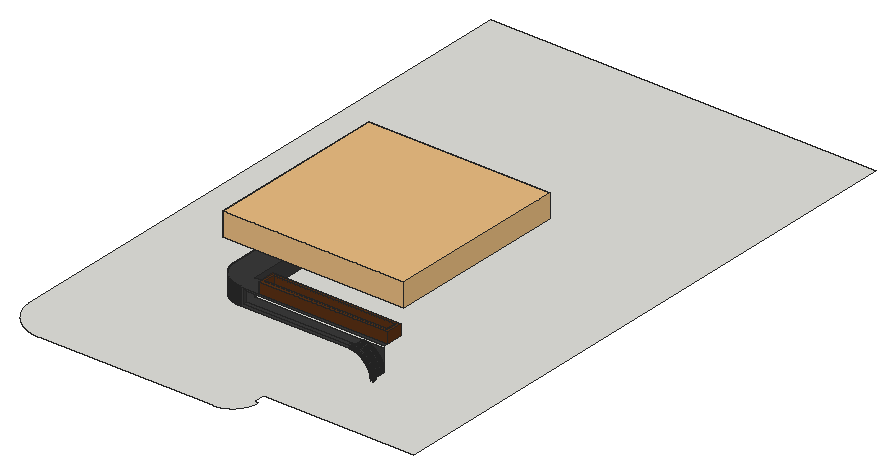
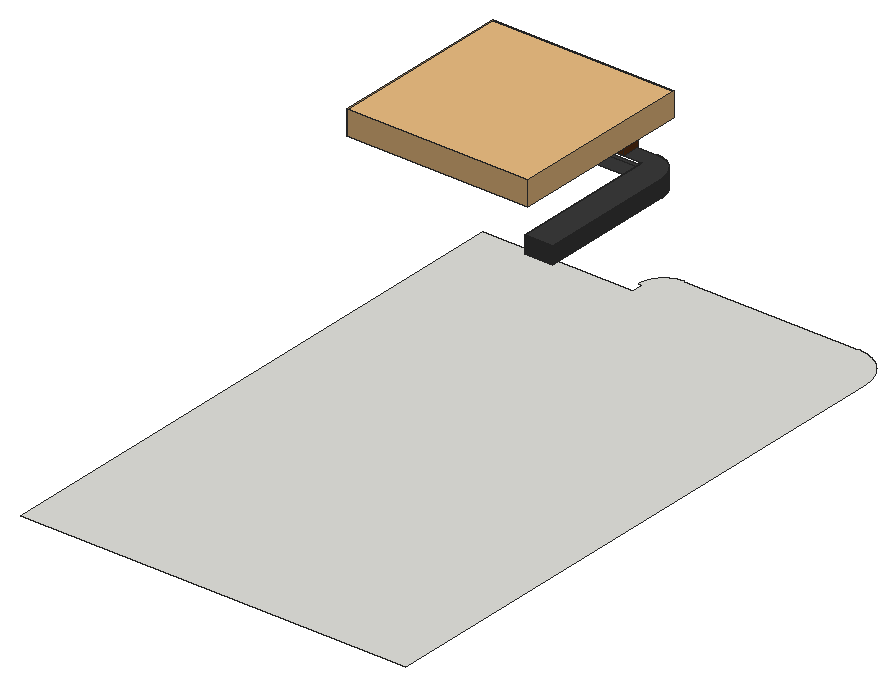
# SketchUp Ruby script. Lengths in inches.
U = 1.inch
M = Sketchup.active_model
def pt(a) = Geom::Point3d.new(a.map { |v| v * U })
def face(e, loops, mat)
  f = e.add_face(loops[0].map { |a| pt(a) })
  loops[1..].each { |l| e.add_face(l.map { |a| pt(a) }).erase! }
  f.material = f.back_material = mat if mat
  f
end
# faces: each face lists its corners as indices into pts; further lists are holes
def faces(e, pts, list, mat = nil) = list.each { |f| face(e, (f[0].is_a?(Array) ? f : [f]).map { |l| l.map { |i| pts[i] } }, mat) }
# xy, xz, yz: faces in a plane at the given z, y or x. An outline is a flat list of corners, or four numbers for a rectangle; further outlines are holes
def ring(l) = l.size == 4 ? [[l[0], l[1]], [l[2], l[1]], [l[2], l[3]], [l[0], l[3]]] : l.each_slice(2).to_a
def flat(e, list, mat, &to3) = list.each { |f| face(e, (f[0].is_a?(Array) ? f : [f]).map { |l| ring(l).map { |u, v| to3.(u, v) } }, mat) }
def xy(e, z, list, mat = nil) = flat(e, list, mat) { |x, y| [x, y, z] }
def xz(e, y, list, mat = nil) = flat(e, list, mat) { |x, z| [x, y, z] }
def yz(e, x, list, mat = nil) = flat(e, list, mat) { |y, z| [x, y, z] }
def lines(e, pts, list) = list.each { |a, b| e.add_line(pt(pts[a]), pt(pts[b])) }
# prism: a flat outline (further loops are holes) pulled along v
def prism(e, loops, v, mat = nil)
  f = face(e, loops, mat); d = Geom::Vector3d.new(v.map { |x| x * U })
  f.pushpull(f.normal.samedirection?(d) ? d.length : -d.length)
end
def box(e, o, s, mat = nil) = prism(e, [[o, [o[0] + s[0], o[1], o[2]], [o[0] + s[0], o[1] + s[1], o[2]], [o[0], o[1] + s[1], o[2]]]], [0, 0, s[2]], mat)
def at(x, y, z, deg = 0) = Geom::Transformation.translation(pt([x, y, z])) * Geom::Transformation.rotation(ORIGIN, Z_AXIS, deg.degrees)
def axes(o, x, y, z) = Geom::Transformation.new([*x, 0, *y, 0, *z, 0, *pt(o).to_a, 1])
def part(name) = M.definitions.add(name)
# library, detail: a bought-in or finely detailed component or shape, given as its bounding box
def library(name, o, s) = part(name).tap { |d| box(d.entities, o, s) }
def detail(e, o, s) = box(e.add_group.entities, o, s)
def put(e, d, t, mat = nil) = e.add_instance(d, t).tap { |i| i.material = mat if mat }
def group(e, t, mat = nil) = e.add_group.tap { |g| g.transformation = t; g.material = mat if mat }.entities
root = M.entities
M.materials.add("1496 AP 8293 CARBON COPY").color = [58, 58, 58]
M.materials.add("[Wood Cherry Original]").color = [91, 49, 20]
c1 = library("Group\#14",[-14,-14.57,-7.55],[148,148.57,19.55])
xy(root,273,[[43.57,64,185.27,64,185.55,64.01,185.82,64.02,186.1,64.03,186.375,64.04,186.65,64.06,186.92,64.09,187.2,64.12,187.74,64.18,188.01,64.22,188.29,64.26,188.56,64.3,189.1,64.4,189.37,64.46,189.63,64.52,189.9,64.58,190.44,64.72,190.96,64.86,191.23,64.94,191.49,65.03,191.75,65.11,192.01,65.2,192.27,65.3,192.53,65.39,192.78,65.49,193.04,65.6,193.79,65.93,194.29,66.17,194.53,66.29,194.78,66.42,195.02,66.54,195.26,66.68,195.5,66.8125,195.74,66.95,195.97,67.09,196.21,67.24,196.4375,67.39,196.67,67.54,196.89,67.69,197.12,67.85,197.56,68.17,198.22,68.68,198.43,68.85,198.85,69.21,199.05,69.39,199.25,69.58,199.46,69.77,199.65,69.96,199.85,70.15,200.04,70.35,200.23,70.54,200.42,70.75,200.61,70.95,200.79,71.15,201.15,71.57,201.32,71.78,201.83,72.44,202.15,72.88,202.31,73.11,202.46,73.33,202.61,73.5625,202.76,73.79,202.91,74.03,203.05,74.26,203.1875,74.5,203.32,74.74,203.46,74.98,203.58,75.22,203.71,75.47,203.83,75.71,204.07,76.21,204.4,76.96,204.51,77.22,204.61,77.47,204.7,77.73,204.8,77.99,204.89,78.25,204.97,78.51,205.06,78.77,205.14,79.04,205.28,79.56,205.42,80.1,205.48,80.37,205.54,80.63,205.6,80.9,205.7,81.44,205.74,81.71,205.78,81.99,205.82,82.26,205.88,82.8,205.91,83.08,205.94,83.35,205.96,83.625,205.97,83.9,205.98,84.18,205.99,84.45,206,84.73,206,85,203,85,203,94,326,94,326,567,11,567,11,96.57,11.01,96.14,11.03,95.7,11.07,94.84,11.1,94.41,11.18,93.55,11.28,92.69,11.34,92.26,11.41,91.84,11.48,91.41,11.55,90.99,11.63,90.5625,11.72,90.14,11.8125,89.72,11.91,89.3,12.02,88.875,12.125,88.46,12.24,88.04,12.36,87.63,12.48,87.21,12.62,86.8,12.75,86.39,12.89,85.98,13.04,85.58,13.19,85.17,13.51,84.37,13.68,83.97,13.85,83.58,14.03,83.18,14.21,82.79,14.4,82.4,14.6,82.02,14.8,81.63,15,81.25,15.42,80.5,15.86,79.76,16.09,79.39,16.32,79.03,16.5625,78.67,16.8,78.31,17.05,77.95,17.3,77.6,17.56,77.26,17.82,76.91,18.08,76.57,18.35,76.23,18.91,75.57,19.1875,75.24,19.48,74.92,19.77,74.6,20.0625,74.28,20.36,73.97,20.67,73.67,20.97,73.36,21.28,73.0625,21.6,72.77,21.92,72.48,22.24,72.1875,22.57,71.91,23.23,71.35,23.57,71.08,23.91,70.82,24.26,70.56,24.6,70.3,24.95,70.05,25.31,69.8,25.67,69.5625,26.03,69.32,26.39,69.09,26.76,68.86,27.5,68.42,28.25,68,28.63,67.8,29.02,67.6,29.4,67.4,29.79,67.21,30.18,67.03,30.58,66.85,30.97,66.68,31.37,66.51,32.17,66.19,32.58,66.04,32.98,65.89,33.39,65.75,33.8,65.62,34.21,65.48,34.63,65.36,35.04,65.24,35.46,65.125,35.875,65.02,36.3,64.91,36.72,64.8125,37.14,64.72,37.5625,64.63,37.99,64.55,38.41,64.48,38.84,64.41,39.26,64.34,39.69,64.28,40.55,64.18,41.41,64.1,41.84,64.07,42.7,64.03,43.14,64.01]])
xy(root,348.99,[[291.47,71,291.71,85]],"1496 AP 8293 CARBON COPY")
xy(root,349,[[202.76,71,202.52,71.01,202.28,71.01,201.8,71.03,201.56,71.05,201.32,71.0625,201.08,71.08,200.84,71.1,200.36,71.15,199.88,71.21,199.64,71.25,199.4,71.28,199.16,71.32,198.93,71.36,198.69,71.41,198.45,71.45,198.22,71.5,197.98,71.55,197.75,71.61,197.51,71.66,197.05,71.78,196.81,71.85,196.58,71.91,196.12,72.05,195.66,72.2,195.4375,72.28,195.21,72.36,194.98,72.44,194.76,72.53,194.53,72.62,194.31,72.7,194.09,72.8,193.87,72.89,193.43,73.09,193.21,73.1875,192.99,73.29,192.77,73.4,192.56,73.51,192.34,73.62,191.92,73.84,191.29,74.2,191.09,74.33,190.88,74.45,190.68,74.58,190.47,74.71,190.27,74.84,190.07,74.98,189.875,75.11,189.68,75.25,189.48,75.39,189.29,75.54,189.09,75.68,188.71,75.98,188.53,76.125,188.34,76.28,188.15,76.43,187.43,77.07,187.26,77.23,187.08,77.4,186.4,78.08,186.23,78.26,186.07,78.43,185.43,79.15,185.28,79.34,185.125,79.53,184.98,79.71,184.68,80.09,184.54,80.29,184.39,80.48,184.25,80.68,184.11,80.875,183.98,81.07,183.84,81.27,183.71,81.47,183.58,81.68,183.45,81.88,183.33,82.09,183.2,82.29,182.84,82.92,182.62,83.34,182.51,83.56,182.4,83.77,182.29,83.99,182.1875,84.21,182.09,84.43,181.89,84.87,181.8,85.09,181.7,85.31,181.62,85.53,181.53,85.76,181.44,85.98,181.36,86.21,181.28,86.4375,181.2,86.66,181.05,87.12,180.91,87.58,180.85,87.81,180.78,88.05,180.66,88.51,180.61,88.75,180.55,88.98,180.5,89.22,180.45,89.45,180.41,89.69,180.36,89.93,180.32,90.16,180.28,90.4,180.25,90.64,180.21,90.88,180.15,91.36,180.1,91.84,180.08,92.08,180.0625,92.32,180.05,92.56,180.03,92.8,180.01,93.28,180.01,93.52,180,93.76,180,205,203,205,203,85,291,85,291,71],[291,71,291.24,85]],"1496 AP 8293 CARBON COPY")
xy(root,351,[[205,71,291,74],[291,71,291.26,74]],"1496 AP 8293 CARBON COPY")
xy(root,361,[[205,71,321,74]],"1496 AP 8293 CARBON COPY")
xy(root,363,[[202.76,71,323,71,323,85,203,85,203,205,180,205,180,93.76,180.01,93.52,180.01,93.28,180.03,92.8,180.05,92.56,180.0625,92.32,180.08,92.08,180.1,91.84,180.15,91.36,180.21,90.88,180.25,90.64,180.28,90.4,180.32,90.16,180.36,89.93,180.41,89.69,180.45,89.45,180.5,89.22,180.55,88.98,180.61,88.75,180.66,88.51,180.78,88.05,180.85,87.81,180.91,87.58,181.05,87.12,181.2,86.66,181.28,86.4375,181.36,86.21,181.44,85.98,181.53,85.76,181.62,85.53,181.7,85.31,181.8,85.09,181.89,84.87,182.09,84.43,182.1875,84.21,182.29,83.99,182.4,83.77,182.51,83.56,182.62,83.34,182.84,82.92,183.2,82.29,183.33,82.09,183.45,81.88,183.58,81.68,183.71,81.47,183.84,81.27,183.98,81.07,184.11,80.875,184.25,80.68,184.39,80.48,184.54,80.29,184.68,80.09,184.98,79.71,185.125,79.53,185.28,79.34,185.43,79.15,186.07,78.43,186.23,78.26,186.4,78.08,187.08,77.4,187.26,77.23,187.43,77.07,188.15,76.43,188.34,76.28,188.53,76.125,188.71,75.98,189.09,75.68,189.29,75.54,189.48,75.39,189.68,75.25,189.875,75.11,190.07,74.98,190.27,74.84,190.47,74.71,190.68,74.58,190.88,74.45,191.09,74.33,191.29,74.2,191.92,73.84,192.34,73.62,192.56,73.51,192.77,73.4,192.99,73.29,193.21,73.1875,193.43,73.09,193.87,72.89,194.09,72.8,194.31,72.7,194.53,72.62,194.76,72.53,194.98,72.44,195.21,72.36,195.4375,72.28,195.66,72.2,196.12,72.05,196.58,71.91,196.81,71.85,197.05,71.78,197.51,71.66,197.75,71.61,197.98,71.55,198.22,71.5,198.45,71.45,198.69,71.41,198.93,71.36,199.16,71.32,199.4,71.28,199.64,71.25,199.88,71.21,200.36,71.15,200.84,71.1,201.08,71.08,201.32,71.0625,201.56,71.05,201.8,71.03,202.28,71.01,202.52,71.01]],"1496 AP 8293 CARBON COPY")
xz(root,71,[[202.76,349,203,363]],"1496 AP 8293 CARBON COPY")
xz(root,71.01,[[202.28,349,202.52,363]],"1496 AP 8293 CARBON COPY")
xz(root,85,[[309,331,309,331.24,308.99,331.47,308.99,331.71,308.98,331.94,308.96,332.18,308.94,332.41,308.92,332.65,308.9,332.88,308.875,333.12,308.85,333.35,308.8125,333.58,308.78,333.82,308.7,334.28,308.65,334.51,308.61,334.74,308.56,334.97,308.5,335.2,308.45,335.43,308.39,335.66,308.32,335.89,308.26,336.11,308.19,336.34,308.12,336.5625,308.04,336.79,307.97,337.01,307.89,337.23,307.8,337.45,307.72,337.67,307.54,338.11,307.44,338.32,307.35,338.54,307.25,338.75,307.14,338.96,307.04,339.17,306.82,339.59,306.7,339.8,306.59,340,306.35,340.4,306.22,340.61,306.1,340.8,305.97,341,305.83,341.2,305.7,341.39,305.5625,341.58,305.42,341.77,305.28,341.96,305.14,342.14,304.99,342.33,304.84,342.51,304.6875,342.69,304.53,342.87,304.375,343.04,304.22,343.22,304.06,343.39,303.89,343.56,303.73,343.73,303.56,343.89,303.39,344.06,303.22,344.22,303.04,344.375,302.87,344.53,302.69,344.6875,302.51,344.84,302.33,344.99,302.14,345.14,301.96,345.28,301.77,345.42,301.58,345.5625,301.39,345.7,301.2,345.83,301,345.97,300.8,346.1,300.61,346.22,300.4,346.35,300,346.59,299.8,346.7,299.59,346.82,299.17,347.04,298.96,347.14,298.75,347.25,298.54,347.35,298.32,347.44,298.11,347.54,297.67,347.72,297.45,347.8,297.23,347.89,297.01,347.97,296.79,348.04,296.5625,348.12,296.34,348.19,296.11,348.26,295.89,348.32,295.66,348.39,295.43,348.45,295.2,348.5,294.97,348.56,294.74,348.61,294.51,348.65,294.28,348.7,293.82,348.78,293.58,348.8125,293.35,348.85,293.12,348.875,292.88,348.9,292.65,348.92,292.41,348.94,292.18,348.96,291.94,348.98,291.71,348.99,291.47,348.99,291.24,349,291,349,309,349]],"1496 AP 8293 CARBON COPY")
xz(root,205,[[180,349,203,363]],"1496 AP 8293 CARBON COPY")
yz(root,180,[[93.76,349,94,363],[94,349,205,363]],"1496 AP 8293 CARBON COPY")
yz(root,180.01,[[93.28,349,93.52,363]],"1496 AP 8293 CARBON COPY")
yz(root,203,[[85,349,205,363]],"1496 AP 8293 CARBON COPY")
yz(root,205,[[71,351,74,361]],"1496 AP 8293 CARBON COPY")
yz(root,308.99,[[71,331.47,85,331.71]],"1496 AP 8293 CARBON COPY")
yz(root,309,[[71,331,85,331.24]],"1496 AP 8293 CARBON COPY")
yz(root,311,[[71,331,74,331.26]],"1496 AP 8293 CARBON COPY")
p = [[309,71,331.24],[308.99,71,331.47],[308.99,85,331.47],[309,85,331.24],[310.99,71,331.52],[311,71,331.26],
  [311,74,331.26],[310.99,74,331.52],[310.98,71,331.79],[310.98,74,331.79],[308.99,71,331.71],[308.98,71,331.94],
  [308.98,85,331.94],[308.99,85,331.71],[310.97,71,332.05],[310.97,74,332.05],[308.96,71,332.18],[308.96,85,332.18],
  [310.96,71,332.31],[310.96,74,332.31],[308.94,71,332.41],[308.94,85,332.41],[310.9375,71,332.57],[310.9375,74,332.57],
  [308.92,71,332.65],[308.92,85,332.65],[308.9,71,332.88],[308.9,85,332.88],[310.92,71,332.83],[310.92,74,332.83],
  [310.89,71,333.09],[310.89,74,333.09],[308.875,71,333.12],[308.875,85,333.12],[308.85,71,333.35],[308.85,85,333.35],
  [310.86,71,333.35],[310.86,74,333.35],[308.8125,71,333.58],[308.8125,85,333.58],[310.83,71,333.61],[310.83,74,333.61],
  [308.78,71,333.82],[308.78,85,333.82],[310.79,71,333.87],[310.79,74,333.87],[308.74,71,334.05],[308.74,85,334.05],
  [310.75,71,334.13],[310.75,74,334.13],[308.7,71,334.28],[308.7,85,334.28],[310.71,71,334.39],[310.71,74,334.39],
  [308.65,71,334.51],[308.65,85,334.51],[310.67,71,334.64],[310.67,74,334.64],[308.61,71,334.74],[308.61,85,334.74],
  [310.62,71,334.9],[310.62,74,334.9],[308.56,71,334.97],[308.56,85,334.97],[310.5625,71,335.16],[310.5625,74,335.16],
  [308.5,71,335.2],[308.5,85,335.2],[308.45,71,335.43],[308.45,85,335.43],[310.51,71,335.41],[310.51,74,335.41],
  [308.39,71,335.66],[308.39,85,335.66],[310.45,71,335.67],[310.45,74,335.67],[308.32,71,335.89],[308.32,85,335.89],
  [310.38,71,335.92],[310.38,74,335.92],[308.26,71,336.11],[308.26,85,336.11],[310.32,71,336.18],[310.32,74,336.18],
  [308.19,71,336.34],[308.19,85,336.34],[310.25,71,336.43],[310.25,74,336.43],[308.12,71,336.5625],[308.12,85,336.5625],
  [310.18,71,336.68],[310.18,74,336.68],[308.04,71,336.79],[308.04,85,336.79],[310.1,71,336.93],[310.1,74,336.93],
  [307.97,71,337.01],[307.97,85,337.01],[310.02,71,337.18],[310.02,74,337.18],[307.89,71,337.23],[307.89,85,337.23],
  [307.8,71,337.45],[307.8,85,337.45],[309.9375,71,337.43],[309.9375,74,337.43],[309.85,71,337.68],[309.85,74,337.68],
  [307.72,71,337.67],[307.72,85,337.67],[307.63,71,337.89],[307.63,85,337.89],[309.76,71,337.92],[309.76,74,337.92],
  [307.54,71,338.11],[307.54,85,338.11],[309.67,71,338.17],[309.67,74,338.17],[307.44,71,338.32],[307.44,85,338.32],
  [309.58,71,338.41],[309.58,74,338.41],[307.35,71,338.54],[307.35,85,338.54],[309.48,71,338.65],[309.48,74,338.65],
  [307.25,71,338.75],[307.25,85,338.75],[307.14,71,338.96],[307.14,85,338.96],[309.375,71,338.89],[309.375,74,338.89],
  [309.27,71,339.13],[309.27,74,339.13],[307.04,71,339.17],[307.04,85,339.17],[309.16,71,339.375],[309.16,74,339.375],
  [306.93,71,339.38],[306.93,85,339.38],[306.82,71,339.59],[306.82,85,339.59],[309.05,71,339.61],[309.05,74,339.61],
  [306.7,71,339.8],[306.7,85,339.8],[308.9375,71,339.85],[308.9375,74,339.85],[306.59,71,340],[306.59,85,340],
  [308.82,71,340.08],[308.82,74,340.08],[306.47,71,340.2],[306.47,85,340.2],[308.7,71,340.3125],[308.7,74,340.3125],
  [306.35,71,340.4],[306.35,85,340.4],[308.58,71,340.54],[308.58,74,340.54],[306.22,71,340.61],[306.22,85,340.61],
  [308.45,71,340.77],[308.45,74,340.77],[306.1,71,340.8],[306.1,85,340.8],[305.97,71,341],[305.97,85,341],
  [308.32,71,341],[308.32,74,341],[305.83,71,341.2],[305.83,85,341.2],[308.1875,71,341.23],[308.1875,74,341.23],
  [305.7,71,341.39],[305.7,85,341.39],[308.05,71,341.45],[308.05,74,341.45],[305.5625,71,341.58],[305.5625,85,341.58],
  [307.91,71,341.67],[307.91,74,341.67],[305.42,71,341.77],[305.42,85,341.77],[307.77,71,341.89],[307.77,74,341.89],
  [305.28,71,341.96],[305.28,85,341.96],[307.63,71,342.11],[307.63,74,342.11],[305.14,71,342.14],[305.14,85,342.14],
  [304.99,71,342.33],[304.99,85,342.33],[307.48,71,342.33],[307.48,74,342.33],[304.84,71,342.51],[304.84,85,342.51],
  [307.33,71,342.54],[307.33,74,342.54],[304.6875,71,342.69],[304.6875,85,342.69],[307.18,71,342.76],[307.18,74,342.76],
  [304.53,71,342.87],[304.53,85,342.87],[307.03,71,342.97],[307.03,74,342.97],[304.375,71,343.04],[304.375,85,343.04],
  [304.22,71,343.22],[304.22,85,343.22],[306.87,71,343.18],[306.87,74,343.18],[304.06,71,343.39],[304.06,85,343.39],
  [306.71,71,343.38],[306.71,74,343.38],[303.89,71,343.56],[303.89,85,343.56],[306.54,71,343.59],[306.54,74,343.59],
  [303.73,71,343.73],[303.73,85,343.73],[306.375,71,343.79],[306.375,74,343.79],[303.56,71,343.89],[303.56,85,343.89],
  [306.21,71,343.99],[306.21,74,343.99],[303.39,71,344.06],[303.39,85,344.06],[306.04,71,344.1875],[306.04,74,344.1875],
  [303.22,71,344.22],[303.22,85,344.22],[303.04,71,344.375],[303.04,85,344.375],[305.86,71,344.38],[305.86,74,344.38],
  [302.87,71,344.53],[302.87,85,344.53],[305.6875,71,344.58],[305.6875,74,344.58],[302.69,71,344.6875],[302.69,85,344.6875],
  [305.51,71,344.77],[305.51,74,344.77],[302.51,71,344.84],[302.51,85,344.84],[302.33,71,344.99],[302.33,85,344.99],
  [305.33,71,344.96],[305.33,74,344.96],[302.14,71,345.14],[302.14,85,345.14],[305.14,71,345.14],[305.14,74,345.14],
  [301.96,71,345.28],[301.96,85,345.28],[304.96,71,345.33],[304.96,74,345.33],[301.77,71,345.42],[301.77,85,345.42],
  [304.77,71,345.51],[304.77,74,345.51],[301.58,71,345.5625],[301.58,85,345.5625],[304.58,71,345.6875],[304.58,74,345.6875],
  [301.39,71,345.7],[301.39,85,345.7],[301.2,71,345.83],[301.2,85,345.83],[304.38,71,345.86],[304.38,74,345.86],
  [301,71,345.97],[301,85,345.97],[304.1875,71,346.04],[304.1875,74,346.04],[300.8,71,346.1],[300.8,85,346.1],
  [303.99,71,346.21],[303.99,74,346.21],[300.61,71,346.22],[300.61,85,346.22],[300.4,71,346.35],[300.4,85,346.35],
  [303.79,71,346.375],[303.79,74,346.375],[300.2,71,346.47],[300.2,85,346.47],[303.59,71,346.54],[303.59,74,346.54],
  [300,71,346.59],[300,85,346.59],[303.38,71,346.71],[303.38,74,346.71],[299.8,71,346.7],[299.8,85,346.7],
  [299.59,71,346.82],[299.59,85,346.82],[303.18,71,346.87],[303.18,74,346.87],[299.38,71,346.93],[299.38,85,346.93],
  [299.17,71,347.04],[299.17,85,347.04],[302.97,71,347.03],[302.97,74,347.03],[298.96,71,347.14],[298.96,85,347.14],
  [302.76,71,347.18],[302.76,74,347.18],[298.75,71,347.25],[298.75,85,347.25],[298.54,71,347.35],[298.54,85,347.35],
  [302.54,71,347.33],[302.54,74,347.33],[298.32,71,347.44],[298.32,85,347.44],[302.33,71,347.48],[302.33,74,347.48],
  [298.11,71,347.54],[298.11,85,347.54],[297.89,71,347.63],[297.89,85,347.63],[302.11,71,347.63],[302.11,74,347.63],
  [297.67,71,347.72],[297.67,85,347.72],[301.89,71,347.77],[301.89,74,347.77],[297.45,71,347.8],[297.45,85,347.8],
  [297.23,71,347.89],[297.23,85,347.89],[301.67,71,347.91],[301.67,74,347.91],[297.01,71,347.97],[297.01,85,347.97],
  [301.45,71,348.05],[301.45,74,348.05],[296.79,71,348.04],[296.5625,71,348.12],[296.5625,85,348.12],[296.79,85,348.04],
  [296.34,71,348.19],[296.34,85,348.19],[301.23,71,348.1875],[301.23,74,348.1875],[296.11,71,348.26],[296.11,85,348.26],
  [301,71,348.32],[301,74,348.32],[295.89,71,348.32],[295.66,71,348.39],[295.66,85,348.39],[295.89,85,348.32],
  [300.77,71,348.45],[300.77,74,348.45],[295.43,71,348.45],[295.2,71,348.5],[295.2,85,348.5],[295.43,85,348.45],
  [300.54,71,348.58],[300.54,74,348.58],[294.97,71,348.56],[294.97,85,348.56],[294.74,71,348.61],[294.51,71,348.65],
  [294.51,85,348.65],[294.74,85,348.61],[300.3125,71,348.7],[300.3125,74,348.7],[294.05,71,348.74],[293.82,71,348.78],
  [293.82,85,348.78],[294.05,85,348.74],[294.28,71,348.7],[294.28,85,348.7],[300.08,71,348.82],[300.08,74,348.82],
  [293.35,71,348.85],[293.12,71,348.875],[293.12,85,348.875],[293.35,85,348.85],[293.58,71,348.8125],[293.58,85,348.8125],
  [299.85,71,348.9375],[299.85,74,348.9375],[292.41,71,348.94],[292.18,71,348.96],[292.18,85,348.96],[292.41,85,348.94],
  [292.65,71,348.92],[292.65,85,348.92],[292.88,71,348.9],[292.88,85,348.9],[299.61,71,349.05],[299.61,74,349.05],
  [201.56,71.05,363],[201.32,71.0625,363],[201.32,71.0625,349],[201.56,71.05,349],[201.8,71.03,363],[201.8,71.03,349],
  [202.04,71.02,363],[202.04,71.02,349],[202.28,71.01,363],[202.28,71.01,349],[202.76,71,363],[202.52,71.01,363],
  [202.52,71.01,349],[202.76,71,349],[291.47,71,348.99],[291.24,71,349],[291.24,85,349],[291.47,85,348.99],
  [291.94,71,348.98],[291.71,71,348.99],[291.71,85,348.99],[291.94,85,348.98],[200.6,71.125,363],[200.36,71.15,363],
  [200.36,71.15,349],[200.6,71.125,349],[200.84,71.1,363],[200.84,71.1,349],[201.08,71.08,363],[201.08,71.08,349],
  [199.64,71.25,363],[199.4,71.28,363],[199.4,71.28,349],[199.64,71.25,349],[199.88,71.21,363],[199.88,71.21,349],
  [200.12,71.18,363],[200.12,71.18,349],[199.16,71.32,363],[198.93,71.36,363],[198.93,71.36,349],[199.16,71.32,349],
  [198.69,71.41,363],[198.45,71.45,363],[198.45,71.45,349],[198.69,71.41,349],[198.22,71.5,363],[197.98,71.55,363],
  [197.98,71.55,349],[198.22,71.5,349],[197.75,71.61,363],[197.51,71.66,363],[197.51,71.66,349],[197.75,71.61,349],
  [197.28,71.72,363],[197.05,71.78,363],[197.05,71.78,349],[197.28,71.72,349],[196.81,71.85,363],[196.58,71.91,363],
  [196.58,71.91,349],[196.81,71.85,349],[196.35,71.98,363],[196.35,71.98,349],[196.12,72.05,363],[196.12,72.05,349],
  [195.89,72.125,363],[195.66,72.2,363],[195.66,72.2,349],[195.89,72.125,349],[195.4375,72.28,363],[195.4375,72.28,349],
  [195.21,72.36,363],[195.21,72.36,349],[194.98,72.44,363],[194.76,72.53,363],[194.76,72.53,349],[194.98,72.44,349],
  [194.53,72.62,363],[194.53,72.62,349],[194.31,72.7,363],[194.31,72.7,349],[194.09,72.8,363],[194.09,72.8,349],
  [193.87,72.89,363],[193.87,72.89,349],[193.65,72.99,363],[193.65,72.99,349],[193.43,73.09,363],[193.43,73.09,349],
  [193.21,73.1875,363],[193.21,73.1875,349],[192.99,73.29,363],[192.99,73.29,349],[192.77,73.4,363],[192.77,73.4,349],
  [192.56,73.51,363],[192.56,73.51,349],[192.34,73.62,363],[192.34,73.62,349],[192.13,73.73,363],[192.13,73.73,349],
  [191.92,73.84,363],[191.92,73.84,349],[191.71,73.96,363],[191.71,73.96,349],[191.5,74.08,363],[191.5,74.08,349],
  [191.29,74.2,363],[191.29,74.2,349],[191.09,74.33,363],[191.09,74.33,349],[190.88,74.45,363],[190.88,74.45,349],
  [190.68,74.58,363],[190.68,74.58,349],[190.47,74.71,363],[190.47,74.71,349],[190.27,74.84,363],[190.27,74.84,349],
  [190.07,74.98,363],[190.07,74.98,349],[189.875,75.11,363],[189.875,75.11,349],[189.68,75.25,363],[189.68,75.25,349],
  [189.48,75.39,363],[189.48,75.39,349],[189.29,75.54,363],[189.29,75.54,349],[189.09,75.68,363],[189.09,75.68,349],
  [188.9,75.83,363],[188.9,75.83,349],[188.71,75.98,363],[188.71,75.98,349],[188.53,76.125,363],[188.53,76.125,349],
  [188.34,76.28,363],[188.34,76.28,349],[188.15,76.43,363],[188.15,76.43,349],[187.97,76.59,363],[187.97,76.59,349],
  [187.79,76.75,363],[187.79,76.75,349],[187.61,76.91,363],[187.61,76.91,349],[187.43,77.07,363],[187.43,77.07,349],
  [187.26,77.23,363],[187.26,77.23,349],[187.08,77.4,363],[187.08,77.4,349],[186.91,77.57,363],[186.91,77.57,349],
  [186.74,77.74,363],[186.74,77.74,349],[186.57,77.91,363],[186.57,77.91,349],[186.4,78.08,363],[186.4,78.08,349],
  [186.23,78.26,363],[186.23,78.26,349],[186.07,78.43,363],[186.07,78.43,349],[185.91,78.61,363],[185.91,78.61,349],
  [185.75,78.79,363],[185.75,78.79,349],[185.59,78.97,363],[185.59,78.97,349],[185.43,79.15,363],[185.43,79.15,349],
  [185.28,79.34,363],[185.28,79.34,349],[185.125,79.53,363],[185.125,79.53,349],[184.98,79.71,363],[184.98,79.71,349],
  [184.83,79.9,363],[184.83,79.9,349],[184.68,80.09,363],[184.68,80.09,349],[184.54,80.29,363],[184.54,80.29,349],
  [184.39,80.48,363],[184.39,80.48,349],[184.25,80.68,363],[184.25,80.68,349],[184.11,80.875,363],[184.11,80.875,349],
  [183.98,81.07,363],[183.98,81.07,349],[183.84,81.27,363],[183.84,81.27,349],[183.71,81.47,363],[183.71,81.47,349],
  [183.58,81.68,363],[183.58,81.68,349],[183.45,81.88,363],[183.45,81.88,349],[183.33,82.09,363],[183.33,82.09,349],
  [183.2,82.29,363],[183.2,82.29,349],[183.08,82.5,363],[183.08,82.5,349],[182.96,82.71,363],[182.96,82.71,349],
  [182.84,82.92,363],[182.84,82.92,349],[182.73,83.13,363],[182.73,83.13,349],[182.62,83.34,363],[182.62,83.34,349],
  [182.51,83.56,363],[182.51,83.56,349],[182.4,83.77,363],[182.4,83.77,349],[182.29,83.99,363],[182.29,83.99,349],
  [182.1875,84.21,363],[182.1875,84.21,349],[182.09,84.43,363],[182.09,84.43,349],[181.99,84.65,363],[181.99,84.65,349],
  [181.89,84.87,363],[181.89,84.87,349],[181.8,85.09,363],[181.8,85.09,349],[181.7,85.31,363],[181.7,85.31,349],
  [181.62,85.53,363],[181.62,85.53,349],[181.53,85.76,363],[181.53,85.76,349],[181.44,85.98,363],[181.44,85.98,349],
  [181.36,86.21,363],[181.36,86.21,349],[181.28,86.4375,363],[181.28,86.4375,349],[181.2,86.66,363],[181.2,86.66,349],
  [181.125,86.89,363],[181.125,86.89,349],[181.05,87.12,363],[181.05,87.12,349],[180.98,87.35,363],[180.98,87.35,349],
  [180.91,87.58,363],[180.91,87.58,349],[180.85,87.81,363],[180.85,87.81,349],[180.78,88.05,363],[180.78,88.05,349],
  [180.72,88.28,363],[180.72,88.28,349],[180.66,88.51,363],[180.66,88.51,349],[180.61,88.75,363],[180.61,88.75,349],
  [180.55,88.98,363],[180.55,88.98,349],[180.5,89.22,363],[180.5,89.22,349],[180.45,89.45,363],[180.45,89.45,349],
  [180.41,89.69,363],[180.41,89.69,349],[180.36,89.93,363],[180.36,89.93,349],[180.32,90.16,363],[180.32,90.16,349],
  [180.28,90.4,363],[180.28,90.4,349],[180.25,90.64,363],[180.25,90.64,349],[180.21,90.88,363],[180.21,90.88,349],
  [180.18,91.12,363],[180.18,91.12,349],[180.15,91.36,363],[180.15,91.36,349],[180.125,91.6,363],[180.125,91.6,349],
  [180.1,91.84,363],[180.1,91.84,349],[180.08,92.08,363],[180.08,92.08,349],[180.0625,92.32,363],[180.0625,92.32,349],
  [180.05,92.56,363],[180.05,92.56,349],[180.03,92.8,363],[180.03,92.8,349],[180.02,93.04,363],[180.02,93.04,349],
  [180.01,93.28,363],[180.01,93.28,349],[180.01,93.52,363],[180,93.76,363],[180,93.76,349],[180.01,93.52,349],
  [299.375,71,349.16],[299.375,74,349.16],[299.13,71,349.27],[299.13,74,349.27],[298.89,71,349.375],[298.89,74,349.375],
  [298.65,71,349.48],[298.65,74,349.48],[298.41,71,349.58],[298.41,74,349.58],[298.17,71,349.67],[298.17,74,349.67],
  [297.92,71,349.76],[297.92,74,349.76],[297.68,71,349.85],[297.68,74,349.85],[297.18,71,350.02],[297.43,71,349.9375],
  [297.43,74,349.9375],[297.18,74,350.02],[296.93,71,350.1],[296.93,74,350.1],[296.68,71,350.18],[296.68,74,350.18],
  [296.18,71,350.32],[296.43,71,350.25],[296.43,74,350.25],[296.18,74,350.32],[295.92,71,350.38],[295.92,74,350.38],
  [295.41,71,350.51],[295.67,71,350.45],[295.67,74,350.45],[295.41,74,350.51],[295.16,71,350.5625],[295.16,74,350.5625],
  [294.64,71,350.67],[294.9,71,350.62],[294.9,74,350.62],[294.64,74,350.67],[294.13,71,350.75],[294.39,71,350.71],
  [294.39,74,350.71],[294.13,74,350.75],[293.35,71,350.86],[293.61,71,350.83],[293.61,74,350.83],[293.35,74,350.86],
  [293.87,71,350.79],[293.87,74,350.79],[292.31,71,350.96],[292.57,71,350.9375],[292.57,74,350.9375],[292.31,74,350.96],
  [292.83,71,350.92],[292.83,74,350.92],[293.09,71,350.89],[293.09,74,350.89],[291.26,71,351],[291.52,71,350.99],
  [291.52,74,350.99],[291.26,74,351],[291.79,71,350.98],[291.79,74,350.98],[292.05,71,350.97],[292.05,74,350.97]]
faces(root,p,[[0,1,2,3],[4,5,6,7],[8,4,7,9],[10,11,12,13],[14,8,9,15],[11,16,17,12],[18,14,15,19],[16,20,21,17],
  [22,18,19,23],[20,24,25,21],[24,26,27,25],[28,22,23,29],[30,28,29,31],[26,32,33,27],[32,34,35,33],[36,30,31,37],
  [34,38,39,35],[40,36,37,41],[38,42,43,39],[44,40,41,45],[42,46,47,43],[48,44,45,49],[46,50,51,47],[52,48,49,53],
  [50,54,55,51],[56,52,53,57],[54,58,59,55],[60,56,57,61],[58,62,63,59],[64,60,61,65],[62,66,67,63],[66,68,69,67],
  [70,64,65,71],[68,72,73,69],[74,70,71,75],[72,76,77,73],[78,74,75,79],[76,80,81,77],[82,78,79,83],[80,84,85,81],
  [86,82,83,87],[84,88,89,85],[90,86,87,91],[88,92,93,89],[94,90,91,95],[92,96,97,93],[98,94,95,99],[96,100,101,97],
  [100,102,103,101],[104,98,99,105],[106,104,105,107],[102,108,109,103],[108,110,111,109],[112,106,107,113],[110,114,115,111],[116,112,113,117],
  [114,118,119,115],[120,116,117,121],[118,122,123,119],[124,120,121,125],[122,126,127,123],[126,128,129,127],[130,124,125,131],[132,130,131,133],
  [128,134,135,129],[136,132,133,137],[134,138,139,135],[138,140,141,139],[142,136,137,143],[140,144,145,141],[146,142,143,147],[144,148,149,145],
  [150,146,147,151],[148,152,153,149],[154,150,151,155],[152,156,157,153],[158,154,155,159],[156,160,161,157],[162,158,159,163],[160,164,165,161],
  [164,166,167,165],[168,162,163,169],[166,170,171,167],[172,168,169,173],[170,174,175,171],[176,172,173,177],[174,178,179,175],[180,176,177,181],
  [178,182,183,179],[184,180,181,185],[182,186,187,183],[188,184,185,189],[186,190,191,187],[190,192,193,191],[194,188,189,195],[192,196,197,193],
  [198,194,195,199],[196,200,201,197],[202,198,199,203],[200,204,205,201],[206,202,203,207],[204,208,209,205],[208,210,211,209],[212,206,207,213],
  [210,214,215,211],[216,212,213,217],[214,218,219,215],[220,216,217,221],[218,222,223,219],[224,220,221,225],[222,226,227,223],[228,224,225,229],
  [226,230,231,227],[232,228,229,233],[230,234,235,231],[234,236,237,235],[238,232,233,239],[236,240,241,237],[242,238,239,243],[240,244,245,241],
  [246,242,243,247],[244,248,249,245],[248,250,251,249],[252,246,247,253],[250,254,255,251],[256,252,253,257],[254,258,259,255],[260,256,257,261],
  [258,262,263,259],[264,260,261,265],[262,266,267,263],[268,264,265,269],[266,270,271,267],[270,272,273,271],[274,268,269,275],[272,276,277,273],
  [278,274,275,279],[276,280,281,277],[282,278,279,283],[280,284,285,281],[284,286,287,285],[288,282,283,289],[286,290,291,287],[292,288,289,293],
  [290,294,295,291],[296,292,293,297],[294,298,299,295],[298,300,301,299],[302,296,297,303],[300,304,305,301],[304,306,307,305],[308,302,303,309],
  [306,310,311,307],[312,308,309,313],[310,314,315,311],[314,316,317,315],[318,312,313,319],[316,320,321,317],[322,318,319,323],[320,324,325,321],
  [324,326,327,325],[328,322,323,329],[326,330,331,327],[332,328,329,333],[330,334,335,331],[334,336,337,335],[338,332,333,339],[336,340,341,337],
  [342,338,339,343],[344,345,346,347],[340,344,347,341],[345,348,349,346],[350,342,343,351],[348,352,353,349],[354,350,351,355],[356,357,358,359],
  [352,356,359,353],[360,354,355,361],[362,363,364,365],[357,362,365,358],[366,360,361,367],[363,368,369,364],[370,371,372,373],[368,370,373,369],
  [374,366,367,375],[376,377,378,379],[380,376,379,381],[371,380,381,372],[382,374,375,383],[384,385,386,387],[388,384,387,389],[377,388,389,378],
  [390,382,383,391],[392,393,394,395],[396,392,395,397],[398,396,397,399],[385,398,399,386],[400,390,391,401],[402,403,404,405],[406,402,405,407],
  [408,406,407,409],[410,408,409,411],[412,413,414,415],[416,417,418,419],[420,421,422,423],[393,420,423,394],[424,425,426,427],[428,424,427,429],
  [430,428,429,431],[403,430,431,404],[432,433,434,435],[436,432,435,437],[438,436,437,439],[425,438,439,426],[440,441,442,443],[433,440,443,434],
  [444,445,446,447],[441,444,447,442],[448,449,450,451],[445,448,451,446],[452,453,454,455],[449,452,455,450],[456,457,458,459],[453,456,459,454],
  [460,461,462,463],[457,460,463,458],[461,464,465,462],[464,466,467,465],[468,469,470,471],[466,468,471,467],[469,472,473,470],[472,474,475,473],
  [476,477,478,479],[474,476,479,475],[477,480,481,478],[480,482,483,481],[482,484,485,483],[484,486,487,485],[486,488,489,487],[488,490,491,489],
  [490,492,493,491],[492,494,495,493],[494,496,497,495],[496,498,499,497],[498,500,501,499],[500,502,503,501],[502,504,505,503],[504,506,507,505],
  [506,508,509,507],[508,510,511,509],[510,512,513,511],[512,514,515,513],[514,516,517,515],[516,518,519,517],[518,520,521,519],[520,522,523,521],
  [522,524,525,523],[524,526,527,525],[526,528,529,527],[528,530,531,529],[530,532,533,531],[532,534,535,533],[534,536,537,535],[536,538,539,537],
  [538,540,541,539],[540,542,543,541],[542,544,545,543],[544,546,547,545],[546,548,549,547],[548,550,551,549],[550,552,553,551],[552,554,555,553],
  [554,556,557,555],[556,558,559,557],[558,560,561,559],[560,562,563,561],[562,564,565,563],[564,566,567,565],[566,568,569,567],[568,570,571,569],
  [570,572,573,571],[572,574,575,573],[574,576,577,575],[576,578,579,577],[578,580,581,579],[580,582,583,581],[582,584,585,583],[584,586,587,585],
  [586,588,589,587],[588,590,591,589],[590,592,593,591],[592,594,595,593],[594,596,597,595],[596,598,599,597],[598,600,601,599],[600,602,603,601],
  [602,604,605,603],[604,606,607,605],[606,608,609,607],[608,610,611,609],[610,612,613,611],[612,614,615,613],[614,616,617,615],[616,618,619,617],
  [618,620,621,619],[620,622,623,621],[622,624,625,623],[624,626,627,625],[626,628,629,627],[628,630,631,629],[630,632,633,631],[632,634,635,633],
  [634,636,637,635],[636,638,639,637],[638,640,641,639],[640,642,643,641],[642,644,645,643],[644,646,647,645],[646,648,649,647],[648,650,651,649],
  [650,652,653,651],[652,654,655,653],[654,656,657,655],[656,658,659,657],[658,660,661,659],[660,662,663,661],[662,664,665,663],[664,666,667,665],
  [666,668,669,667],[668,670,671,669],[670,672,673,671],[672,674,675,673],[674,676,677,675],[676,678,679,677],[678,680,681,679],[680,682,683,681],
  [682,684,685,683],[684,686,687,685],[686,688,689,687],[688,690,691,689],[690,692,693,691],[692,694,695,693],[694,696,697,695],[696,698,699,697],
  [698,700,701,699],[700,702,703,701],[704,705,706,707],[708,400,401,709],[710,708,709,711],[712,710,711,713],[714,712,713,715],[716,714,715,717],
  [718,716,717,719],[720,718,719,721],[722,720,721,723],[724,725,726,727],[725,722,723,726],[728,724,727,729],[730,728,729,731],[732,733,734,735],
  [733,730,731,734],[736,732,735,737],[738,739,740,741],[739,736,737,740],[742,738,741,743],[744,745,746,747],[745,742,743,746],[748,749,750,751],
  [749,744,747,750],[752,753,754,755],[753,756,757,754],[756,748,751,757],[758,759,760,761],[759,762,763,760],[762,764,765,763],[764,752,755,765],
  [766,767,768,769],[767,770,771,768],[770,772,773,771],[772,758,761,773]],"1496 AP 8293 CARBON COPY")
g1 = group(root,at(203,71,363),"[Wood Cherry Original]")
xy(g1,0,[[15,0,120,14]])
xy(g1,3,[[17.5,2.5,117.5,11.5]])
xy(g1,9,[[[15,0,120,14],[17.5,2.5,117.5,11.5]]])
xz(g1,0,[[15,0,120,9]])
xz(g1,2.5,[[17.5,3,117.5,9]])
xz(g1,11.5,[[17.5,3,117.5,9]])
xz(g1,14,[[15,0,120,9]])
yz(g1,15,[[0,0,14,9]])
yz(g1,17.5,[[2.5,3,11.5,9]])
yz(g1,117.5,[[2.5,3,11.5,9]])
yz(g1,120,[[0,0,14,9]])
put(root,c1,at(203,85,402),"1496 AP 8293 CARBON COPY")
